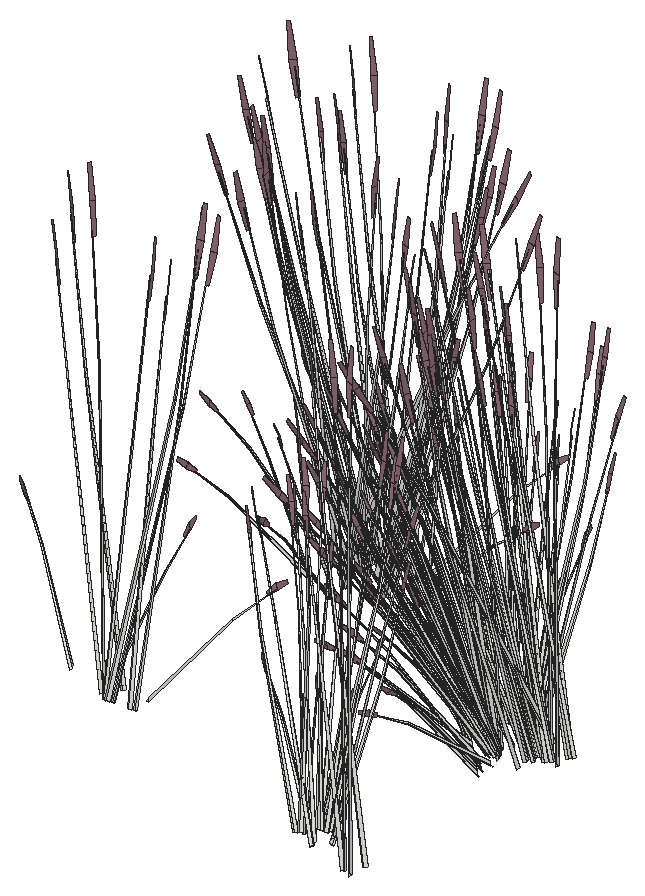
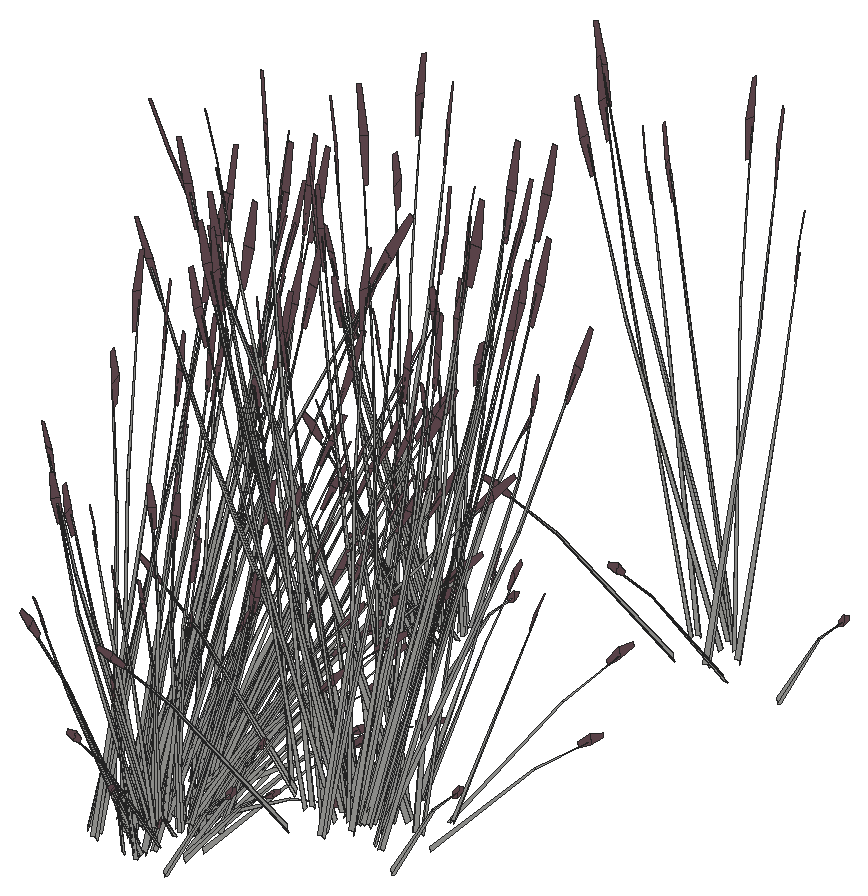
# SketchUp Ruby script. Lengths in inches.
U = 1.inch
M = Sketchup.active_model
def pt(a) = Geom::Point3d.new(a.map { |v| v * U })
def face(e, loops, mat)
  f = e.add_face(loops[0].map { |a| pt(a) })
  loops[1..].each { |l| e.add_face(l.map { |a| pt(a) }).erase! }
  f.material = f.back_material = mat if mat
  f
end
# faces: each face lists its corners as indices into pts; further lists are holes
def faces(e, pts, list, mat = nil) = list.each { |f| face(e, (f[0].is_a?(Array) ? f : [f]).map { |l| l.map { |i| pts[i] } }, mat) }
# xy, xz, yz: faces in a plane at the given z, y or x. An outline is a flat list of corners, or four numbers for a rectangle; further outlines are holes
def ring(l) = l.size == 4 ? [[l[0], l[1]], [l[2], l[1]], [l[2], l[3]], [l[0], l[3]]] : l.each_slice(2).to_a
def flat(e, list, mat, &to3) = list.each { |f| face(e, (f[0].is_a?(Array) ? f : [f]).map { |l| ring(l).map { |u, v| to3.(u, v) } }, mat) }
def xy(e, z, list, mat = nil) = flat(e, list, mat) { |x, y| [x, y, z] }
def xz(e, y, list, mat = nil) = flat(e, list, mat) { |x, z| [x, y, z] }
def yz(e, x, list, mat = nil) = flat(e, list, mat) { |y, z| [x, y, z] }
def lines(e, pts, list) = list.each { |a, b| e.add_line(pt(pts[a]), pt(pts[b])) }
# prism: a flat outline (further loops are holes) pulled along v
def prism(e, loops, v, mat = nil)
  f = face(e, loops, mat); d = Geom::Vector3d.new(v.map { |x| x * U })
  f.pushpull(f.normal.samedirection?(d) ? d.length : -d.length)
end
def box(e, o, s, mat = nil) = prism(e, [[o, [o[0] + s[0], o[1], o[2]], [o[0] + s[0], o[1] + s[1], o[2]], [o[0], o[1] + s[1], o[2]]]], [0, 0, s[2]], mat)
def at(x, y, z, deg = 0) = Geom::Transformation.translation(pt([x, y, z])) * Geom::Transformation.rotation(ORIGIN, Z_AXIS, deg.degrees)
def axes(o, x, y, z) = Geom::Transformation.new([*x, 0, *y, 0, *z, 0, *pt(o).to_a, 1])
def part(name) = M.definitions.add(name)
# library, detail: a bought-in or finely detailed component or shape, given as its bounding box
def library(name, o, s) = part(name).tap { |d| box(d.entities, o, s) }
def detail(e, o, s) = box(e.add_group.entities, o, s)
def put(e, d, t, mat = nil) = e.add_instance(d, t).tap { |i| i.material = mat if mat }
def group(e, t, mat = nil) = e.add_group.tap { |g| g.transformation = t; g.material = mat if mat }.entities
root = M.entities
M.materials.add("LightPink_Translucent").color = [144, 107, 117]
c1 = part("blade")
p = [[2.15,0.21,22],[0,0.17,0],[0.09,0.45,0],[2.18,0.31,22],[2.29,0.31,22],[0.38,0.45,0],
  [2.48,0.24,33],[2.49,0.24,33],[2.48,0.22,33]]
faces(c1.entities,p,[[0,1,2,3],[4,5,2,3],[6,3,4,7],[8,0,3,6]])
c2 = part("seeds")
p = [[0.3,-0.1,1.38],[-0.01,-0.03,1.59],[-0.01,-0.03,0.03],[0.14,-0.07,-0.07],[0.29,-0.03,3],[0.15,0.01,3.11]]
faces(c2.entities,p,[[0,1,2,3],[1,0,4,5]],"LightPink_Translucent")
c3 = part("blade with seeds")
put(c3.entities,c1,at(0,0,0))
put(c3.entities,c2,axes([2.4,0.25,30.99],[1.5799,-0.05474,1.17369],[-0.12525,1.92788,0.29478],[-0.07173,-0.02425,1.56792]))
put(root,c3,axes([36.41,436.9375,43.49],[0.16438,0.10347,1.76342],[0.27873,0.95868,-0.26939],[-0.36432,0.20444,0.30037]))
put(root,c3,axes([43.1,471.63,43.49],[0.03108,0.16322,1.76342],[-0.62654,0.85237,-0.26939],[-0.44504,-0.04296,0.30037]))
put(root,c3,axes([43.11,434.75,44.06],[-0.82544,0.77843,-0.62353],[-1.0254,-0.70586,-0.16365],[-0.33076,0.19418,1.37633]))
put(root,c3,axes([42.76,476.2,43.49],[0.16438,0.10347,1.76342],[0.27873,0.95868,-0.26939],[-0.36432,0.20444,0.30037]))
put(root,c3,axes([44.47,436.875,44.02],[-1.14694,0.51783,-0.49651],[-0.68554,-0.92854,0],[-0.26122,0.11794,1.57504]))
put(root,c3,axes([47.2,473.11,44.06],[-1.27479,-0.1698,-0.62353],[0.26901,-1.04736,-0.16365],[-0.38043,-0.12691,1.37633]))
put(root,c3,axes([44.01,433.85,44.67],[0.1428,1.18174,-0.29095],[-1.48733,0.07145,-0.50002],[-0.26191,0.15741,1.59708]))
put(root,c3,axes([45.53,475.09,44.02],[-1.14694,-0.51783,-0.49651],[0.68554,-0.92854,0],[-0.26122,-0.11794,1.57504]))
put(root,c3,axes([45.02,467.38,43.49],[-0.11871,0.13643,1.76342],[-1.19964,0.29415,-0.26939],[-0.2898,-0.26759,0.30037]))
put(root,c3,axes([44.28,467.9,44.13],[-0.35352,0.84566,-0.03893],[-1.08806,-0.26014,-0.17649],[-0.1652,-0.13832,0.58215]))
put(root,c3,axes([48.64,473.26,44.67],[-1.23732,0.68758,-0.29095],[-0.8228,-0.97154,-0.50002],[-0.30528,-0.09867,1.59708]))
put(root,c3,axes([45.84,474.71,44.03],[-0.28787,-0.90242,-0.30978],[1.14332,-0.25625,0.30978],[-0.23049,-0.10406,1.38974]))
put(root,c3,axes([49.47,474.02,44.06],[-0.82544,0.77843,-0.62353],[-1.0254,-0.70586,-0.16365],[-0.33076,0.19418,1.37633]))
put(root,c3,axes([41.48,437.03,43.49],[0.19833,-0.05635,1.76342],[1.19302,0.31018,-0.26939],[0.03489,0.3496,0.30037]))
put(root,c3,axes([50.03,473.58,44.46],[-1.19666,-0.83357,-0.25192],[1.00694,-0.93603,0.5513],[-0.32224,0.09751,1.68216]))
put(root,c3,axes([47.86,472.78,44.21],[-0.73619,-0.86927,-0.44739],[1.11511,-0.61213,0.21531],[-0.23824,-0.10756,1.43643]))
put(root,c3,axes([49.43,473.4,44.21],[-1.33077,0.06393,-0.44739],[-0.12035,-1.06125,0.21531],[-0.23824,0.10756,1.43643]))
put(root,c3,axes([44.55,433.39,44.21],[-0.59459,0.93321,-0.44739],[-1.23546,-0.44912,0.21531],[0,0.21512,1.43643]))
put(root,c3,axes([47.97,473.28,44.4375],[0.32481,-1.2272,-0.23429],[1.54007,0.21392,0.51271],[-0.26911,-0.16947,1.5644]))
put(root,c3,axes([50.83,476.14,44.02],[-1.14694,0.51783,-0.49651],[-0.68554,-0.92854,0],[-0.26122,0.11794,1.57504]))
put(root,c3,axes([44.03,470.98,44.02],[0,-1.03566,-0.49651],[1.37109,0,0],[0,-0.23588,1.57504]))
put(root,c3,axes([50.56,475.73,44.03],[-1.14332,-0.25625,-0.30978],[0.28787,-0.90242,0.30978],[-0.23049,0.10406,1.38974]))
put(root,c3,axes([47.62,472.18,44.67],[-1.38012,-0.49416,-0.29095],[0.66454,-1.04299,-0.50002],[-0.04337,-0.25608,1.59708]))
put(root,c3,axes([50.36,473.11,44.67],[0.1428,1.18174,-0.29095],[-1.48733,0.07145,-0.50002],[-0.26191,0.15741,1.59708]))
put(root,c3,axes([47,471.13,44.1],[-0.50328,-1.06202,-0.69835],[1.44974,-0.38248,-0.18329],[-0.05563,-0.35963,1.54149]))
put(root,c3,axes([44.62,471,44.03],[0.85545,-0.64616,-0.30978],[0.85545,0.64616,0.30978],[0,-0.20813,1.38974]))
put(root,c3,axes([48.49,466.82,44.13],[-0.84686,0.59414,-0.03893],[-0.77596,-0.65071,-0.17649],[-0.05463,-0.18438,0.58215]))
put(root,c3,axes([47.69,433.79,44.03],[-0.85545,0.64616,-0.30978],[-0.85545,-0.64616,0.30978],[0,0.20813,1.38974]))
put(root,c3,axes([45.25,433.67,44.09],[0.44936,0.94823,-0.69212],[-1.29441,0.3415,-0.18165],[0.04967,0.32109,1.52773]))
put(root,c3,axes([44.7,432.61,44.67],[1.38012,0.49416,-0.29095],[-0.66454,1.04299,-0.50002],[0.04337,0.25608,1.59708]))
put(root,c3,axes([48.28,433.81,44.02],[0,1.03566,-0.49651],[-1.37109,0,0],[0,0.23588,1.57504]))
put(root,c3,axes([48.7,466.1,43.49],[-0.20555,0.03731,1.76342],[-1.13672,-0.42002,-0.26939],[0.01907,-0.35034,0.30037]))
put(root,c3,axes([47.77,471.4,44.21],[0.59459,-0.93321,-0.44739],[1.23546,0.44912,0.21531],[0,-0.21512,1.43643]))
put(root,c3,axes([50.9,472.65,44.21],[-0.59459,0.93321,-0.44739],[-1.23546,-0.44912,0.21531],[0,0.21512,1.43643]))
put(root,c3,axes([54.05,473.05,44.03],[-0.85545,0.64616,-0.30978],[-0.85545,-0.64616,0.30978],[0,0.20813,1.38974]))
put(root,c3,axes([51.6,472.93,44.09],[0.44936,0.94823,-0.69212],[-1.29441,0.3415,-0.18165],[0.04967,0.32109,1.52773]))
put(root,c3,axes([48.31,470.94,44.67],[-0.1428,-1.18174,-0.29095],[1.48733,-0.07145,-0.50002],[0.26191,-0.15741,1.59708]))
put(root,c3,axes([46.73,437.0625,43.49],[0.08928,-0.14952,1.76342],[1.12407,-0.44035,-0.26939],[0.34078,0.22791,0.30037]))
put(root,c3,axes([51.05,471.875,44.67],[1.38012,0.49416,-0.29095],[-0.66454,1.04299,-0.50002],[0.04337,0.25608,1.59708]))
put(root,c3,axes([48.11,468.32,44.03],[1.14332,0.25625,-0.30978],[-0.28787,0.90242,0.30978],[0.23049,-0.10406,1.38974]))
put(root,c3,axes([54.63,473.07,44.02],[0,1.03566,-0.49651],[-1.37109,0,0],[0,0.23588,1.57504]))
put(root,c3,axes([47.84,467.91,44.02],[1.14694,-0.51783,-0.49651],[0.68554,0.92854,0],[0.26122,-0.11794,1.57504]))
put(root,c3,axes([50.79,474.29,44.18],[1.2866,-0.3514,-0.19198],[0.45209,1.01223,0.00008],[0.14202,-0.03884,1.73897]))
put(root,c3,axes([50.8125,471.28,44.21],[0.73619,0.86927,-0.44739],[-1.11511,0.61213,0.21531],[0.23824,0.10756,1.43643]))
put(root,c3,axes([49.2,470.04,44.06],[0.82544,-0.77843,-0.62353],[1.0254,0.70586,-0.16365],[0.33076,-0.19418,1.37633]))
put(root,c3,axes([52.83,469.35,44.03],[0.28787,0.90242,-0.30978],[-1.14332,0.25625,0.30978],[0.23049,0.10406,1.38974]))
put(root,c3,axes([69.75,465.24,34.25],[0.50831,-0.02346,1.71376],[-0.33721,1.01661,0.13857],[-0.72439,-0.06288,0.73262]))
put(root,c3,axes([50.03,470.79,44.67],[1.23732,-0.68758,-0.29095],[0.8228,0.97154,-0.50002],[0.30528,0.09867,1.59708]))
put(root,c3,axes([46.9,470.18,43.59],[-1.20625,0.41464,1.28929],[-0.38394,-1.1897,0.50096],[0.74071,0.01979,1.46642]))
put(root,c3,axes([69.96,467.03,34.25],[0.42521,-0.21906,1.71376],[0.35798,1.01226,0.13857],[-0.66754,0.22878,0.73262]))
put(root,c3,axes([68.64,468.75,32.97],[0.42589,0.08502,1.43002],[0.2745,0.86839,-0.30754],[-0.57851,0.16255,0.61141]))
put(root,c3,axes([53.73,467.88,43.49],[-0.18342,-0.08159,1.76342],[-0.47115,-0.9115,-0.26939],[0.31784,-0.24736,0.30037]))
put(root,c3,axes([72.41,465.97,33.72],[0.34834,-0.14982,1.77064],[0.12012,1.04605,0.13857],[-0.75452,0.1388,0.63284]))
put(root,c3,axes([53.14,468.96,44.02],[1.14694,0.51783,-0.49651],[-0.68554,0.92854,0],[0.26122,0.11794,1.57504]))
put(root,c3,axes([53.09,476.33,43.49],[0.08928,-0.14952,1.76342],[1.12407,-0.44035,-0.26939],[0.34078,0.22791,0.30037]))
put(root,c3,axes([68.66,466.67,35.09],[-0.20012,0.13446,1.74944],[0.01702,0.98243,-0.27667],[-0.45871,0.12776,0.14031]))
put(root,c3,axes([71.27,464.29,35.36],[-1.22504,-0.02494,-0.71045],[0.08228,-1.05005,0.08574],[-0.51899,-0.11081,1.00501]))
put(root,c3,axes([51.47,470.94,44.06],[1.27479,0.1698,-0.62353],[-0.26901,1.04736,-0.16365],[0.38043,0.12691,1.37633]))
put(root,c3,axes([56.9,471.56,44.26],[-0.75977,-0.66224,-0.06488],[0.83212,-0.6068,-0.29416],[0.23578,-0.04272,0.97024]))
put(root,c3,axes([70.29,464.55,32.97],[0.23927,0.28834,1.43002],[-0.55135,0.78376,-0.30754],[-0.56612,-0.18733,0.61141]))
put(root,c3,axes([69.31,466.11,34.9],[-1.01846,-0.28891,-0.35414],[0.29705,-0.84289,0.4572],[-0.41005,0.07729,0.87481]))
put(root,c3,axes([70.71,463.61,34.25],[0.45521,0.17844,1.71376],[-0.94204,0.74856,0.13857],[-0.58713,-0.33769,0.73262]))
put(root,c3,axes([66.4375,467.67,35.08],[0.1564,0.02778,1.77383],[0.48382,0.91506,-0.16761],[-0.32016,0.24017,0.31391]))
put(root,c3,axes([70,466.54,35.06],[-0.332,0.94205,-0.51099],[-1.13828,-0.3229,-0.3958],[-0.45829,0.08638,0.97773]))
put(root,c3,axes([70.87,464.51,35.06],[-0.88986,0.68603,-0.51099],[-0.77932,-0.72471,-0.3958],[-0.45212,-0.10438,0.97773]))
put(root,c3,axes([69.43,466.48,31.87],[0.03108,0.16322,1.76342],[-0.62654,0.85237,-0.26939],[-0.44504,-0.04296,0.30037]))
put(root,c3,axes([69.61,462.58,35.08],[0.09085,0.10335,1.77383],[-0.43798,0.92907,-0.16761],[-0.44357,0.00672,0.31391]))
put(root,c3,axes([67.75,470.57,33.14],[0.51072,-0.46938,1.1486],[0.20153,0.74307,0.84392],[-0.36908,0.13305,0.25299]))
put(root,c3,axes([70.625,461.96,35.09],[-0.26368,-0.00731,1.74944],[-0.83946,0.73103,-0.27667],[-0.44791,-0.14937,0.14031]))
put(root,c3,axes([69.54,466.01,35.11],[0.34623,-0.9443,0.48003],[1.13828,0.3229,0.3958],[-0.44763,0.05675,0.9933]))
put(root,c3,axes([69.95,465.74,35.41],[0.6166,0.93779,-0.1216],[-1.09436,0.46085,-0.67495],[-0.46117,0.12373,1.02557]))
put(root,c3,axes([71.33,463.79,35.41],[-0.06562,1.05324,-0.1216],[-1.2424,-0.02879,-0.67495],[-0.4785,-0.07316,1.02557]))
put(root,c3,axes([70.54,463.86,34.9],[-0.69728,-0.64842,-0.35414],[0.79619,-0.61382,0.4572],[-0.40453,-0.09339,0.87481]))
put(root,c3,axes([69.46,465.76,35.11],[-0.4501,-0.70615,0.0643],[0.82077,-0.34564,0.50621],[-0.36181,0.0682,0.77189]))
put(root,c3,axes([71.52,433.14,36.3],[0.30609,-0.31822,1.71376],[0.77286,0.85893,0.13857],[-0.53009,0.39116,0.73262]))
put(root,c3,axes([71.52,467.71,34.25],[0.30609,-0.31822,1.71376],[0.77286,0.85893,0.13857],[-0.53009,0.39116,0.73262]))
put(root,c3,axes([69.68,433.98,36.95],[-1.06674,0.14801,-0.35414],[-0.28168,-0.84611,0.4572],[-0.30569,0.22726,0.87481]))
put(root,c3,axes([69.68,468.54,34.9],[-1.06674,0.14801,-0.35414],[-0.28168,-0.84611,0.4572],[-0.30569,0.22726,0.87481]))
put(root,c3,axes([69.1,436.49,33.92],[0.16438,0.10347,1.76342],[0.27873,0.95868,-0.26939],[-0.36432,0.20444,0.30037]))
put(root,c3,axes([69.1,471.05,31.87],[0.16438,0.10347,1.76342],[0.27873,0.95868,-0.26939],[-0.36432,0.20444,0.30037]))
put(root,c3,axes([68.86,465.41,33.14],[0.78239,-0.07411,1.1486],[-0.49629,0.65296,0.84392],[-0.38663,-0.09795,0.25299]))
put(root,c3,axes([69.82,468.36,35.11],[-0.30393,-0.95317,0.48003],[1.19224,-0.16542,0.3958],[-0.35138,0.22417,0.9933]))
put(root,c3,axes([70.43,463.62,35.47],[1.01205,-0.7643,0.53763],[0.87284,0.81167,0.4433],[-0.47482,-0.14098,1.11249]))
put(root,c3,axes([69.58,468.18,35.11],[-0.8413,-0.43556,0.0643],[0.48981,-0.62025,0.50621],[-0.26973,0.20053,0.77189]))
put(root,c3,axes([71.29,433.93,36.3],[0.22818,-0.35597,1.71376],[0.95725,0.73667,0.13857],[-0.43183,0.45914,0.73262]))
put(root,c3,axes([71.29,468.49,34.25],[0.22818,-0.35597,1.71376],[0.95725,0.73667,0.13857],[-0.43183,0.45914,0.73262]))
put(root,c3,axes([70.38,466.02,35.43],[1.01846,0.28891,0.35414],[-0.29705,0.84289,-0.4572],[-0.41005,0.07729,0.87481]))
put(root,c3,axes([56.32,471.79,43.49],[-0.06405,-0.15723,1.76342],[0.44421,-0.91974,-0.26939],[0.4481,-0.01323,0.30037]))
put(root,c3,axes([70.56,434.08,37.11],[0.31482,0.94565,-0.51099],[-1.19224,0.16542,-0.3958],[-0.34166,0.254,0.97773]))
put(root,c3,axes([70.56,468.64,35.06],[0.31482,0.94565,-0.51099],[-1.19224,0.16542,-0.3958],[-0.34166,0.254,0.97773]))
put(root,c3,axes([70.89,463.61,35.11],[0.06171,-0.78753,0.0643],[0.9318,0.02159,0.50621],[-0.35694,-0.08241,0.77189]))
put(root,c3,axes([68.7,435.77,37.14],[-0.03046,0.20495,1.74944],[0.86449,0.71297,-0.27667],[-0.22632,0.33716,0.14031]))
put(root,c3,axes([68.7,470.34,35.09],[-0.03046,0.20495,1.74944],[0.86449,0.71297,-0.27667],[-0.22632,0.33716,0.14031]))
put(root,c3,axes([73.53,467.96,32.44],[-1.27479,-0.1698,-0.62353],[0.26901,-1.04736,-0.16365],[-0.38043,-0.12691,1.37633]))
put(root,c3,axes([73.76,462.25,35.81],[-0.81789,0.99285,-0.13619],[-1.18445,-0.572,-0.75594],[-0.41173,-0.28051,1.14864]))
put(root,c3,axes([71.53,464.2,35.43],[0.69728,0.64842,0.35414],[-0.79619,0.61382,-0.4572],[-0.40453,-0.09339,0.87481]))
put(root,c3,axes([73.4,463.06,35.36],[-1.04497,-0.50058,-0.71045],[0.74264,-0.8772,0.08574],[-0.3786,-0.29889,1.00501]))
put(root,c3,axes([72.91,463.08,35.06],[-1.20928,0.24619,-0.51099],[-0.21154,-0.93233,-0.3958],[-0.32481,-0.26718,0.97773]))
put(root,c3,axes([71.86,469.94,32.39],[-1.14694,-0.51783,-0.49651],[0.68554,-0.92854,0],[-0.26122,-0.11794,1.57504]))
put(root,c3,axes([71.35,462.23,31.87],[-0.11871,0.13643,1.76342],[-1.19964,0.29415,-0.26939],[-0.2898,-0.26759,0.30037]))
put(root,c3,axes([70,433.4,37.46],[1.1336,0.57106,-0.1216],[-0.65308,0.827,-0.67495],[-0.32027,0.28747,1.02557]))
put(root,c3,axes([70,467.96,35.41],[1.1336,0.57106,-0.1216],[-0.65308,0.827,-0.67495],[-0.32027,0.28747,1.02557]))
put(root,c3,axes([72.56,470.57,32.75],[-0.7662,1.03778,0],[-1.28187,-0.57875,-0.51607],[-0.29196,-0.13181,1.63711]))
put(root,c3,axes([68.125,435.88,38.07],[1.08141,0.27645,-0.06488],[-0.33265,0.85086,-0.29416],[-0.17688,0.12919,0.97024]))
put(root,c3,axes([68.125,470.44,36.02],[1.08141,0.27645,-0.06488],[-0.33265,0.85086,-0.29416],[-0.17688,0.12919,0.97024]))
put(root,c3,axes([70.55,468.04,35.43],[1.06674,-0.14801,0.35414],[0.28168,0.84611,-0.4572],[-0.30569,0.22726,0.87481]))
put(root,c3,axes([71.16,437.51,35.02],[0.38672,-0.16338,1.43002],[0.95481,0.49262,-0.30754],[-0.28419,0.42626,0.61141]))
put(root,c3,axes([71.16,472.07,32.97],[0.38672,-0.16338,1.43002],[0.95481,0.49262,-0.30754],[-0.28419,0.42626,0.61141]))
put(root,c3,axes([70.61,462.76,32.5],[-0.35352,0.84566,-0.03893],[-1.08806,-0.26014,-0.17649],[-0.1652,-0.13832,0.58215]))
put(root,c3,axes([73.44,459.89,35.08],[-0.02286,0.12414,1.77383],[-1.12758,0.45052,-0.16761],[-0.33182,-0.23029,0.31391]))
put(root,c3,axes([72.23,461.69,32.97],[-0.07421,0.33879,1.43002],[-1.08488,0.28361,-0.30754],[-0.25359,-0.4379,0.61141]))
put(root,c3,axes([72.59,462.57,34.25],[0.28013,0.33252,1.71376],[-1.29445,0.27994,0.13857],[-0.29256,-0.52202,0.73262]))
put(root,c3,axes([74.98,468.12,33.04],[-1.23732,0.68758,-0.29095],[-0.8228,-0.97154,-0.50002],[-0.30528,-0.09867,1.59708]))
put(root,c3,axes([71.56,435.72,37.16],[-0.87265,-0.70663,0.48003],[0.92674,-0.60943,0.3958],[-0.16097,0.33153,0.9933]))
put(root,c3,axes([71.56,470.29,35.11],[-0.87265,-0.70663,0.48003],[0.92674,-0.60943,0.3958],[-0.16097,0.33153,0.9933]))
put(root,c3,axes([73.04,462.39,34.9],[-0.18927,-0.83419,-0.35414],[1.08199,-0.22027,0.4572],[-0.29062,-0.23905,0.87481]))
put(root,c3,axes([70.02,466.62,32.75],[-1.53239,0,0],[0,-1.1575,-0.51607],[0,-0.26363,1.63711]))
put(root,c3,axes([72.18,469.56,32.4],[-0.28787,-0.90242,-0.30978],[1.14332,-0.25625,0.30978],[-0.23049,-0.10406,1.38974]))
put(root,c3,axes([71.24,435.66,37.16],[-1.00708,-0.04826,0.0643],[0.02761,-0.72867,0.50621],[-0.10538,0.27912,0.77189]))
put(root,c3,axes([71.24,470.22,35.11],[-1.00708,-0.04826,0.0643],[0.02761,-0.72867,0.50621],[-0.10538,0.27912,0.77189]))
put(root,c3,axes([71.55,435.94,36.95],[-0.82919,0.54528,-0.35414],[-0.78493,-0.62262,0.4572],[-0.11943,0.31634,0.87481]))
put(root,c3,axes([71.55,470.5,34.9],[-0.82919,0.54528,-0.35414],[-0.78493,-0.62262,0.4572],[-0.11943,0.31634,0.87481]))
put(root,c3,axes([75.8,434.3,34.49],[-0.82544,0.77843,-0.62353],[-1.0254,-0.70586,-0.16365],[-0.33076,0.19418,1.37633]))
put(root,c3,axes([75.8,468.87,32.44],[-0.82544,0.77843,-0.62353],[-1.0254,-0.70586,-0.16365],[-0.33076,0.19418,1.37633]))
put(root,c3,axes([73.68,463.07,35.43],[0.18927,0.83419,0.35414],[-1.08199,0.22027,-0.4572],[-0.29062,-0.23905,0.87481]))
put(root,c3,axes([68.6,437.875,37.14],[0.13903,-0.06253,1.77383],[1.14912,0.41591,-0.16761],[-0.027,0.34629,0.31391]))
put(root,c3,axes([68.6,472.44,35.08],[0.13903,-0.06253,1.77383],[1.14912,0.41591,-0.16761],[-0.027,0.34629,0.31391]))
put(root,c3,axes([71.21,466.3125,32.71],[-1.1399,0.87071,0.30756],[-1.1406,-0.86155,-0.36492],[-0.03981,-0.24727,1.64885]))
put(root,c3,axes([75.9,468.72,33.7],[1.05902,0.41762,1.51261],[-1.03748,0.89969,0.59816],[-0.46471,-0.53324,1.26806]))
put(root,c3,axes([71.86,461.14,33.14],[0.63926,0.36046,1.1486],[-0.93099,0.21668,0.84392],[-0.1992,-0.27702,0.25299]))
put(root,c3,axes([76.37,468.43,32.84],[-1.19666,-0.83357,-0.25192],[1.00694,-0.93603,0.5513],[-0.32224,0.09751,1.68216]))
put(root,c3,axes([74.19,467.63,32.59],[-0.73619,-0.86927,-0.44739],[1.11511,-0.61213,0.21531],[-0.23824,-0.10756,1.43643]))
put(root,c3,axes([72.11,435.36,37.77],[-0.03189,0.95798,-0.7886],[-1.34277,-0.06434,0.09517],[-0.14171,0.40585,1.11556]))
put(root,c3,axes([72.11,469.92,35.71],[-0.03189,0.95798,-0.7886],[-1.34277,-0.06434,0.09517],[-0.14171,0.40585,1.11556]))
put(root,c3,axes([72.08,438.05,35.19],[-0.03171,-0.6158,1.1486],[0.7925,0.43922,0.84392],[-0.15586,0.29352,0.25299]))
put(root,c3,axes([72.08,472.62,33.14],[-0.03171,-0.6158,1.1486],[0.7925,0.43922,0.84392],[-0.15586,0.29352,0.25299]))
put(root,c3,axes([73.2,462.09,35.47],[1.36515,-0.26619,0.53763],[0.23692,1.04421,0.4433],[-0.32106,-0.30775,1.11249]))
put(root,c3,axes([75.76,468.25,32.59],[-1.33077,0.06393,-0.44739],[-0.12035,-1.06125,0.21531],[-0.23824,0.10756,1.43643]))
put(root,c3,axes([73.51,462.32,35.11],[0.55698,-0.6579,0.0643],[0.79316,0.38303,0.50621],[-0.25643,-0.21093,0.77189]))
put(root,c3,axes([73.22,470.03,32.85],[1.14694,0.51783,0.49651],[-0.68554,0.92854,0],[-0.26122,-0.11794,1.57504]))
put(root,c3,axes([71.66,436.71,35.79],[0.02693,-0.53464,1.54345],[1.21102,0.2824,0.21329],[-0.10493,0.5698,0.72882]))
put(root,c3,axes([71.66,471.27,33.74],[0.02693,-0.53464,1.54345],[1.21102,0.2824,0.21329],[-0.10493,0.5698,0.72882]))
put(root,c3,axes([74.3,468.13,32.81],[0.32481,-1.2272,-0.23429],[1.54007,0.21392,0.51271],[-0.26911,-0.16947,1.5644]))
put(root,c3,axes([74.86,468.42,32.99],[-0.23642,0.92427,0.1448],[-1.15506,-0.16044,-0.41347],[-0.21021,-0.09491,1.26744]))
put(root,c3,axes([74.73,460.36,35.09],[-0.18744,-0.14521,1.74944],[-1.25089,0.09206,-0.27667],[-0.19964,-0.34731,0.14031]))
put(root,c3,axes([77.16,436.43,34.45],[-1.14694,0.51783,-0.49651],[-0.68554,-0.92854,0],[-0.26122,0.11794,1.57504]))
put(root,c3,axes([77.16,470.99,32.39],[-1.14694,0.51783,-0.49651],[-0.68554,-0.92854,0],[-0.26122,0.11794,1.57504]))
put(root,c3,axes([70.37,465.83,32.39],[0,-1.03566,-0.49651],[1.37109,0,0],[0,-0.23588,1.57504]))
put(root,c3,axes([70.95,466.79,32.85],[0,1.03566,0.49651],[-1.37109,0,0],[0,-0.23588,1.57504]))
put(root,c3,axes([77.23,470.71,32.57],[-0.75665,-1.04141,-0.05142],[1.28187,-0.57875,0.51607],[-0.31588,0.09915,1.6363]))
put(root,c3,axes([72.38,435.68,37.43],[0.87728,0.69587,-0.5672],[-0.92674,0.60943,-0.43934],[-0.13348,0.35356,1.08528]))
put(root,c3,axes([72.38,470.24,35.38],[0.87728,0.69587,-0.5672],[-0.92674,0.60943,-0.43934],[-0.13348,0.35356,1.08528]))
put(root,c3,axes([76.89,470.58,32.4],[-1.14332,-0.25625,-0.30978],[0.28787,-0.90242,0.30978],[-0.23049,0.10406,1.38974]))
put(root,c3,axes([71.99,435.16,37.48],[0.82919,-0.54528,0.35414],[0.78493,0.62262,-0.4572],[-0.11943,0.31634,0.87481]))
put(root,c3,axes([71.99,469.73,35.43],[0.82919,-0.54528,0.35414],[0.78493,0.62262,-0.4572],[-0.11943,0.31634,0.87481]))
put(root,c3,axes([73.95,467.03,33.04],[-1.38012,-0.49416,-0.29095],[0.66454,-1.04299,-0.50002],[-0.04337,-0.25608,1.59708]))
put(root,c3,axes([77.55,432.16,35.27],[-0.03348,-0.97511,1.41272],[1.51511,0.25277,0.59816],[-0.35835,0.53357,1.3335]))
put(root,c3,axes([77.55,466.72,33.22],[-0.03348,-0.97511,1.41272],[1.51511,0.25277,0.59816],[-0.35835,0.53357,1.3335]))
put(root,c3,axes([71.46,435.3125,37.83],[1.34686,0.05131,-0.13498],[-0.03681,0.97156,-0.74919],[-0.09356,0.37418,1.13838]))
put(root,c3,axes([71.46,469.875,35.77],[1.34686,0.05131,-0.13498],[-0.03681,0.97156,-0.74919],[-0.09356,0.37418,1.13838]))
put(root,c3,axes([71.43,436.72,35.25],[1.11329,-0.1834,0.06507],[0.25594,0.73887,-0.86304],[-0.07058,0.37403,0.7736]))
put(root,c3,axes([71.43,471.29,33.2],[1.11329,-0.1834,0.06507],[0.25594,0.73887,-0.86304],[-0.07058,0.37403,0.7736]))
put(root,c3,axes([76.69,433.4,35.09],[0.1428,1.18174,-0.29095],[-1.48733,0.07145,-0.50002],[-0.26191,0.15741,1.59708]))
put(root,c3,axes([76.69,467.97,33.04],[0.1428,1.18174,-0.29095],[-1.48733,0.07145,-0.50002],[-0.26191,0.15741,1.59708]))
put(root,c3,axes([73.33,465.98,32.47],[-0.50328,-1.06202,-0.69835],[1.44974,-0.38248,-0.18329],[-0.05563,-0.35963,1.54149]))
